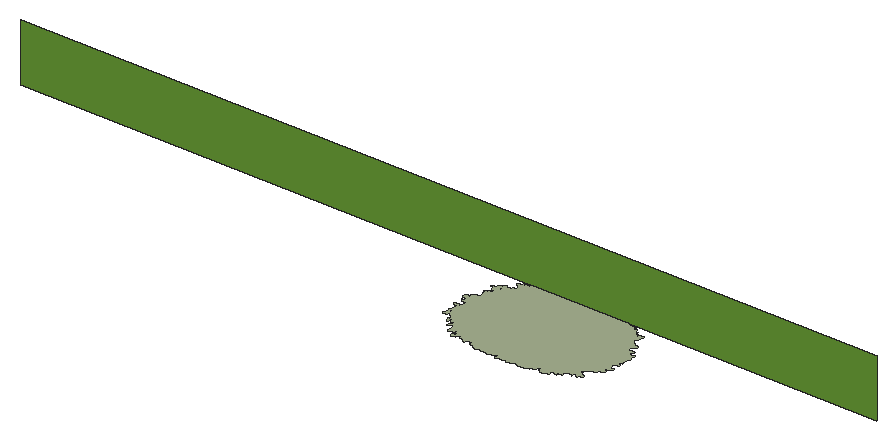
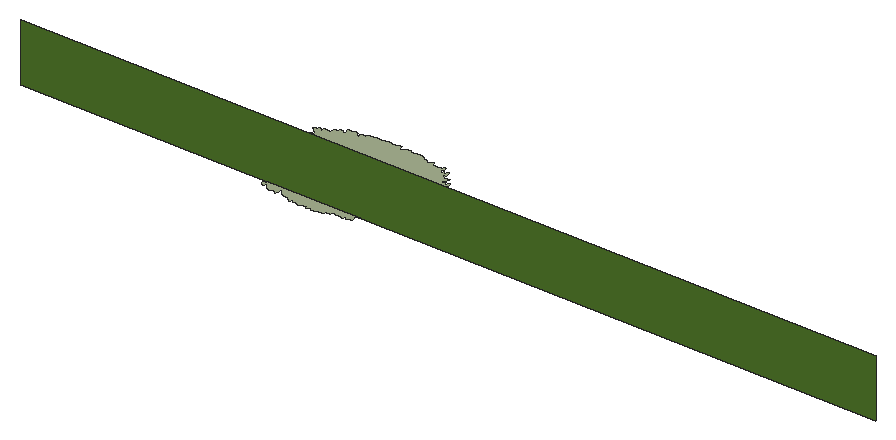
# SketchUp Ruby script. Lengths in inches.
U = 1.inch
M = Sketchup.active_model
def pt(a) = Geom::Point3d.new(a.map { |v| v * U })
def face(e, loops, mat)
  f = e.add_face(loops[0].map { |a| pt(a) })
  loops[1..].each { |l| e.add_face(l.map { |a| pt(a) }).erase! }
  f.material = f.back_material = mat if mat
  f
end
# faces: each face lists its corners as indices into pts; further lists are holes
def faces(e, pts, list, mat = nil) = list.each { |f| face(e, (f[0].is_a?(Array) ? f : [f]).map { |l| l.map { |i| pts[i] } }, mat) }
# xy, xz, yz: faces in a plane at the given z, y or x. An outline is a flat list of corners, or four numbers for a rectangle; further outlines are holes
def ring(l) = l.size == 4 ? [[l[0], l[1]], [l[2], l[1]], [l[2], l[3]], [l[0], l[3]]] : l.each_slice(2).to_a
def flat(e, list, mat, &to3) = list.each { |f| face(e, (f[0].is_a?(Array) ? f : [f]).map { |l| ring(l).map { |u, v| to3.(u, v) } }, mat) }
def xy(e, z, list, mat = nil) = flat(e, list, mat) { |x, y| [x, y, z] }
def xz(e, y, list, mat = nil) = flat(e, list, mat) { |x, z| [x, y, z] }
def yz(e, x, list, mat = nil) = flat(e, list, mat) { |y, z| [x, y, z] }
def lines(e, pts, list) = list.each { |a, b| e.add_line(pt(pts[a]), pt(pts[b])) }
# prism: a flat outline (further loops are holes) pulled along v
def prism(e, loops, v, mat = nil)
  f = face(e, loops, mat); d = Geom::Vector3d.new(v.map { |x| x * U })
  f.pushpull(f.normal.samedirection?(d) ? d.length : -d.length)
end
def box(e, o, s, mat = nil) = prism(e, [[o, [o[0] + s[0], o[1], o[2]], [o[0] + s[0], o[1] + s[1], o[2]], [o[0], o[1] + s[1], o[2]]]], [0, 0, s[2]], mat)
def at(x, y, z, deg = 0) = Geom::Transformation.translation(pt([x, y, z])) * Geom::Transformation.rotation(ORIGIN, Z_AXIS, deg.degrees)
def axes(o, x, y, z) = Geom::Transformation.new([*x, 0, *y, 0, *z, 0, *pt(o).to_a, 1])
def part(name) = M.definitions.add(name)
# library, detail: a bought-in or finely detailed component or shape, given as its bounding box
def library(name, o, s) = part(name).tap { |d| box(d.entities, o, s) }
def detail(e, o, s) = box(e.add_group.entities, o, s)
def put(e, d, t, mat = nil) = e.add_instance(d, t).tap { |i| i.material = mat if mat }
def group(e, t, mat = nil) = e.add_group.tap { |g| g.transformation = t; g.material = mat if mat }.entities
root = M.entities
M.materials.add("Boxwoodplan").color = [166, 177, 144]
M.materials.add("[Grass Dark Green]").color = [106, 157, 55]
xy(root,9.058,[[[215.792,67.129,215.681,67.133,215.586,67.159,215.53,67.215,215.528,67.317,215.554,67.382,215.618,67.445,215.667,67.509,215.725,67.606,215.539,67.635,215.449,67.644,215.469,67.732,215.555,67.79,215.586,67.8,215.581,67.846,215.492,67.877,215.376,67.837,215.279,67.706,215.136,67.551,214.975,67.464,214.87,67.441,214.809,67.416,214.793,67.373,214.649,67.281,214.455,67.251,214.366,67.26,214.286,67.306,214.286,67.328,214.331,67.359,214.422,67.437,214.49,67.483,214.401,67.498,214.288,67.48,214.168,67.436,214.072,67.445,213.975,67.454,213.878,67.447,213.751,67.403,213.551,67.356,213.462,67.349,213.424,67.443,213.416,67.465,213.349,67.473,213.26,67.454,213.091,67.336,212.891,67.328,212.661,67.353,212.494,67.446,212.353,67.61,212.536,67.702,212.436,67.756,212.3,67.772,212.174,67.749,212.102,67.697,212.021,67.672,211.905,67.738,211.863,67.806,211.951,67.847,211.977,67.907,211.982,67.957,211.941,68.009,211.869,68.085,211.783,68.117,211.696,68.064,211.63,68.038,211.574,68.08,211.557,68.103,211.533,68.121,211.504,68.111,211.424,68.058,211.353,68.01,211.277,67.923,211.265,67.79,211.194,67.749,211.144,67.723,211.084,67.725,210.985,67.746,210.898,67.793,210.854,67.861,210.846,67.951,210.855,68.018,210.868,68.04,210.849,68.08,210.635,68.1,210.703,68.135,210.677,68.136,210.584,68.13,210.414,68.146,210.337,68.173,210.32,68.206,210.335,68.224,210.46,68.314,210.458,68.371,210.373,68.393,210.214,68.39,210.083,68.319,209.986,68.233,209.911,68.199,209.864,68.172,209.863,68.154,209.899,68.101,209.883,68.046,209.813,68.081,209.749,68.121,209.688,68.072,209.666,68.017,209.634,67.904,209.587,67.855,209.514,67.822,209.423,67.816,209.353,67.841,209.334,67.874,209.341,67.892,209.362,67.932,209.384,67.991,209.353,68.048,209.252,68.149,209.366,68.229,209.427,68.269,209.507,68.285,209.574,68.315,209.629,68.37,209.714,68.476,209.642,68.503,209.5625,68.511,209.43,68.53,209.392,68.565,209.399,68.584,209.474,68.62,209.636,68.657,209.678,68.709,209.673,68.748,209.647,68.764,209.497,68.711,209.451,68.732,209.452,68.752,209.475,68.814,209.314,68.825,209.233,68.833,209.179,68.826,209.172,68.806,209.156,68.71,209.141,68.642,209.099,68.591,209.052,68.578,209.033,68.594,208.974,68.639,208.929,68.757,208.89,68.783,208.863,68.784,208.809,68.777,208.802,68.757,208.8,68.641,208.746,68.523,208.685,68.449,208.605,68.419,208.526,68.422,208.48,68.448,208.447,68.506,208.447,68.564,208.501,68.677,208.615,68.784,208.635,68.803,208.622,68.823,208.595,68.829,208.515,68.847,208.434,68.86,208.407,68.875,208.414,68.895,208.434,68.914,208.583,68.982,208.745,69.005,208.787,69.108,208.76,69.169,208.713,69.191,208.686,69.187,208.523,69.168,208.482,69.2,208.489,69.22,208.516,69.279,208.674,69.334,208.846,69.403,208.894,69.442,208.881,69.463,208.784,69.436,208.613,69.417,208.469,69.372,208.38,69.386,208.353,69.392,208.359,69.412,208.38,69.426,208.435,69.47,208.407,69.507,208.38,69.503,208.297,69.511,208.242,69.56,208.228,69.601,208.201,69.597,208.118,69.575,207.961,69.489,207.812,69.413,207.738,69.38,207.683,69.392,207.696,69.412,207.715,69.452,207.742,69.469,207.766,69.55,207.816,69.65,207.848,69.759,207.899,69.812,207.972,69.852,208.016,69.972,208.038,70.112,208.058,70.227,208.054,70.285,208.009,70.321,207.928,70.335,207.842,70.335,207.768,70.31,207.758,70.245,207.759,70.184,207.726,70.124,207.638,70.087,207.581,70.096,207.543,70.155,207.532,70.216,207.506,70.337,207.501,70.4,207.46,70.453,207.433,70.475,207.395,70.491,207.336,70.479,207.302,70.46,207.3,70.428,207.292,70.366,207.295,70.229,207.32,70.167,207.312,70.103,207.261,70.038,207.213,70.01,207.175,69.998,207.137,70.003,207.095,70.011,207.077,70.039,207.073,70.166,207.094,70.223,207.139,70.276,207.155,70.306,207.147,70.334,207.09,70.34,207.008,70.346,206.971,70.362,206.948,70.39,206.945,70.453,206.96,70.483,206.995,70.499,207.167,70.472,207.246,70.497,207.295,70.526,207.356,70.573,207.369,70.636,207.346,70.662,207.302,70.664,207.225,70.67,207.133,70.681,207.032,70.717,207.013,70.746,207.019,70.76,207.038,70.763,207.098,70.775,207.273,70.761,207.363,70.787,207.375,70.844,207.349,70.907,207.277,70.946,207.198,70.953,207.085,70.946,206.985,70.921,206.902,70.939,206.898,70.968,206.918,70.997,206.965,71.054,207.031,71.11,207.084,71.19,207.076,71.224,207.031,71.241,206.966,71.24,206.848,71.14,206.808,71.141,206.774,71.161,206.796,71.22,206.812,71.287,206.769,71.35,206.729,71.366,206.709,71.367,206.703,71.352,206.707,71.306,206.704,71.164,206.663,71.102,206.624,71.108,206.589,71.131,206.491,71.262,206.467,71.327,206.442,71.355,206.427,71.344,206.371,71.293,206.336,71.234,206.356,71.103,206.361,71.037,206.341,70.971,206.291,70.962,206.257,70.978,206.247,71.023,206.267,71.155,206.276,71.233,206.276,71.27,206.261,71.282,206.246,71.272,206.167,71.237,206.127,71.183,206.118,71.12,206.079,71.077,205.942,70.987,205.902,70.977,205.858,70.986,205.778,71.026,205.758,71.056,205.762,71.089,205.795,71.151,205.892,71.237,205.982,71.263,206.072,71.263,206.167,71.267,206.106,71.318,205.955,71.404,205.938,71.466,205.991,71.503,206.083,71.573,206.202,71.635,206.32,71.709,206.356,71.723,206.382,71.746,206.408,71.789,206.411,71.882,206.444,72.003,206.445,72.065,206.424,72.086,206.402,72.095,206.339,72.109,206.306,72.104,206.302,72.088,206.314,71.996,206.272,71.934,206.224,71.899,206.147,71.871,206.076,71.858,205.915,71.833,205.88,71.839,205.867,71.853,205.867,71.86,205.876,71.901,205.893,71.947,205.935,71.995,206.004,72.042,206.063,72.063,206.121,72.065,206.16,72.068,206.18,72.075,206.203,72.096,206.198,72.121,206.144,72.151,206.076,72.207,206.044,72.264,206.04,72.331,206.053,72.382,206.105,72.426,206.131,72.432,206.142,72.425,206.162,72.411,206.205,72.35,206.254,72.304,206.382,72.226,206.456,72.192,206.491,72.177,206.511,72.184,206.535,72.206,206.542,72.222,206.553,72.263,206.538,72.32,206.495,72.366,206.463,72.389,206.429,72.401,206.369,72.401,206.295,72.404,206.252,72.446,206.166,72.519,206.107,72.569,206.068,72.617,206.069,72.646,206.093,72.671,206.149,72.698,206.184,72.703,206.225,72.7,206.285,72.679,206.347,72.677,206.383,72.684,206.417,72.726,206.466,72.757,206.525,72.764,206.596,72.764,206.75,72.771,206.89,72.792,206.923,72.808,206.924,72.826,206.918,72.868,206.906,72.913,206.917,72.957,206.947,73.06,206.934,73.083,206.911,73.097,206.854,73.126,206.801,73.164,206.728,73.192,206.655,73.195,206.605,73.184,206.584,73.17,206.559,73.119,206.564,73.098,206.575,73.093,206.599,73.088,206.75,73.076,206.776,73.071,206.781,73.0625,206.772,73.046,206.732,73.007,206.687,72.964,206.622,72.928,206.56,72.884,206.488,72.849,206.451,72.852,206.431,72.863,206.406,72.9,206.399,72.995,206.382,73.02,206.4,73.034,206.406,73.077,206.4,73.088,206.389,73.088,206.374,73.087,206.348,73.083,206.316,73.076,206.298,73.065,206.217,72.97,206.185,72.915,206.154,72.892,206.131,72.895,206.105,72.916,206.096,72.932,206.09,72.973,206.119,73.057,206.124,73.102,206.115,73.13,206.095,73.137,206.057,73.128,206.037,73.114,205.991,73.064,205.869,72.957,205.833,72.932,205.807,72.927,205.77,72.935,205.758,72.951,205.849,73.057,205.912,73.102,205.926,73.129,205.925,73.145,205.916,73.152,205.905,73.148,205.89,73.143,205.859,73.131,205.775,73.108,205.608,73.089,205.535,73.096,205.487,73.121,205.465,73.149,205.464,73.165,205.481,73.217,205.529,73.264,205.589,73.281,205.66,73.284,205.734,73.266,205.862,73.223,205.948,73.197,205.959,73.201,205.959,73.22,205.95,73.239,205.925,73.287,205.924,73.342,205.931,73.407,205.943,73.437,205.96,73.45,206.009,73.413,206.048,73.363,206.075,73.317,206.085,73.255,206.097,73.204,206.112,73.176,206.135,73.175,206.27,73.157,206.343,73.144,206.378,73.14,206.396,73.154,206.411,73.202,206.356,73.244,206.297,73.309,206.28,73.335,206.28,73.352,206.314,73.46,206.344,73.483,206.371,73.489,206.386,73.477,206.395,73.459,206.424,73.414,206.435,73.39,206.447,73.391,206.468,73.404,206.548,73.482,206.565,73.528,206.566,73.579,206.552,73.611,206.531,73.623,206.468,73.646,206.428,73.666,206.42,73.687,206.436,73.736,206.492,73.773,206.526,73.795,206.539,73.816,206.547,73.869,206.545,73.916,206.45,73.992,206.306,74.014,206.244,74.031,206.209,74.013,206.181,74.014,206.112,74.031,206.093,74.058,206.102,74.082,206.228,74.185,206.222,74.217,206.2,74.233,206.155,74.225,206.126,74.216,206,74.154,205.96,74.107,205.911,74.063,205.842,74.049,205.814,74.05,205.767,74.102,205.795,74.126,205.8125,74.165,205.844,74.188,205.938,74.22,205.983,74.25,205.972,74.281,205.959,74.283,205.949,74.276,205.923,74.27,205.884,74.273,205.749,74.284,205.602,74.3125,205.578,74.327,205.584,74.347,205.609,74.375,205.822,74.435,205.885,74.434,205.946,74.419,206.006,74.391,206.033,74.393,206.039,74.403,206.088,74.48,206.112,74.495,206.118,74.515,206.118,74.583,206.107,74.593,206.094,74.591,206.036,74.591,205.979,74.585,205.932,74.568,205.908,74.576,205.887,74.596,205.862,74.63,205.842,74.718,205.853,74.806,205.883,74.848,205.889,74.88,205.902,74.923,205.939,74.944,205.935,74.99,205.913,75.026,205.824,75.003,205.806,74.969,205.807,74.95,205.81,74.886,205.73,74.839,205.589,74.745,205.433,74.7,205.349,74.725,205.307,74.778,205.298,74.904,205.426,74.99,205.509,75.003,205.552,75.027,205.576,75.061,205.575,75.081,205.489,75.112,205.416,75.138,205.354,75.194,205.389,75.249,205.465,75.278,205.561,75.312,205.626,75.311,205.805,75.267,205.897,75.246,205.982,75.25,206.033,75.269,206.039,75.289,206.023,75.355,205.962,75.407,205.917,75.415,205.805,75.485,205.758,75.527,205.744,75.564,205.737,75.617,205.737,75.644,205.75,75.659,205.792,75.695,205.843,75.709,205.957,75.741,205.988,75.751,206.028,75.75,206.078,75.746,206.091,75.733,206.106,75.703,206.12,75.689,206.13,75.689,206.158,75.692,206.174,75.704,206.195,75.754,206.223,75.787,206.239,75.81,206.242,75.835,206.258,75.86,206.278,75.872,206.326,75.884,206.365,75.877,206.386,75.833,206.39,75.781,206.407,75.755,206.428,75.754,206.47,75.796,206.495,75.838,206.509,75.942,206.525,75.968,206.557,75.975,206.589,75.974,206.608,75.963,206.629,75.94,206.661,75.94,206.714,75.961,206.758,76.007,206.772,76.032,206.761,76.046,206.821,76.043,206.85,76.046,206.866,76.066,206.871,76.114,206.905,76.155,206.939,76.2,206.885,76.243,206.818,76.272,206.781,76.271,206.748,76.261,206.706,76.249,206.664,76.255,206.642,76.271,206.621,76.295,206.598,76.397,206.611,76.423,206.616,76.439,206.626,76.443,206.731,76.463,206.777,76.472,206.795,76.483,206.785,76.486,206.699,76.514,206.633,76.526,206.605,76.519,206.57,76.52,206.534,76.52,206.498,76.532,206.46,76.582,206.442,76.611,206.442,76.642,206.457,76.663,206.486,76.678,206.517,76.697,206.525,76.725,206.555,76.782,206.582,76.836,206.588,76.89,206.581,76.917,206.541,76.928,206.463,76.954,206.29,77.001,206.254,77.018,206.237,77.042,206.273,77.097,206.317,77.131,206.363,77.159,206.418,77.178,206.47,77.1875,206.523,77.184,206.578,77.16,206.633,77.162,206.66,77.167,206.673,77.187,206.69,77.228,206.727,77.264,206.748,77.282,206.774,77.284,206.843,77.267,206.905,77.256,206.931,77.253,206.955,77.268,207.042,77.336,207.129,77.401,207.183,77.498,207.179,77.542,207.138,77.579,207.021,77.617,206.895,77.647,206.809,77.719,206.751,77.755,206.682,77.776,206.655,77.788,206.641,77.808,206.663,77.855,206.711,77.896,206.709,77.981,206.659,78.06,206.529,78.116,206.241,78.212,206.22,78.246,206.292,78.31,206.413,78.362,206.518,78.367,206.575,78.353,206.619,78.327,206.668,78.317,206.721,78.326,206.782,78.337,206.811,78.368,206.826,78.448,206.843,78.483,206.897,78.482,206.954,78.471,207.002,78.451,207.069,78.392,207.093,78.358,207.107,78.318,207.108,78.249,207.114,78.245,207.123,78.249,207.15,78.262,207.201,78.268,207.29,78.271,207.37,78.235,207.404,78.17,207.429,78.092,207.499,78.047,207.539,78.035,207.557,78.034,207.584,78.043,207.679,78.05,207.696,78.055,207.676,78.071,207.613,78.095,207.561,78.099,207.523,78.118,207.504,78.152,207.501,78.164,207.504,78.184,207.519,78.191,207.554,78.192,207.596,78.185,207.702,78.156,207.817,78.152,207.869,78.159,207.887,78.162,207.913,78.173,207.869,78.203,207.828,78.213,207.742,78.228,207.684,78.242,207.643,78.244,207.621,78.248,207.596,78.263,207.544,78.289,207.497,78.315,207.475,78.348,207.485,78.404,207.514,78.442,207.555,78.471,207.515,78.502,207.46,78.517,207.417,78.52,207.362,78.528,207.331,78.555,207.313,78.591,207.299,78.6,207.27,78.599,207.154,78.571,207.102,78.557,207.053,78.559,207.005,78.562,206.956,78.578,206.908,78.595,206.868,78.602,206.782,78.65,206.807,78.662,206.809,78.669,206.82,78.709,206.836,78.745,206.862,78.782,206.893,78.814,206.937,78.839,206.99,78.862,207.035,78.873,207.141,78.867,207.218,78.862,207.251,78.858,207.262,78.857,207.262,78.87,207.254,78.912,207.233,78.956,207.197,78.995,207.154,79.026,207.121,79.073,207.123,79.096,207.134,79.117,207.181,79.147,207.233,79.17,207.26,79.169,207.286,79.163,207.34,79.148,207.408,79.142,207.455,79.127,207.479,79.114,207.497,79.095,207.541,79.055,207.58,79.02,207.625,78.989,207.681,78.976,207.735,78.981,207.78,79.01,207.812,79.046,207.861,79.084,207.887,79.083,207.909,79.069,207.95,79.027,207.997,78.994,208.125,79.019,208.199,79.037,208.24,79.065,208.246,79.085,208.225,79.102,208.174,79.124,208.164,79.147,208.172,79.169,208.188,79.214,208.195,79.273,208.199,79.299,208.222,79.315,208.249,79.316,208.279,79.308,208.321,79.288,208.455,79.248,208.516,79.226,208.555,79.193,208.582,79.153,208.597,79.13,208.604,79.123,208.613,79.126,208.621,79.131,208.654,79.176,208.66,79.212,208.65,79.315,208.628,79.362,208.604,79.397,208.569,79.436,208.559,79.466,208.57,79.477,208.581,79.475,208.603,79.476,208.602,79.484,208.607,79.508,208.6,79.549,208.585,79.705,208.587,79.782,208.472,79.802,208.375,79.804,208.3125,79.8125,208.295,79.819,208.281,79.83,208.294,79.839,208.407,79.882,208.441,79.911,208.44,79.924,208.417,79.948,208.381,79.952,208.328,79.94,208.28,79.918,208.263,79.919,208.248,79.945,208.274,80.028,208.277,80.069,208.276,80.082,208.252,80.103,208.163,80.085,208.05,80.088,207.941,80.105,207.88,80.185,207.878,80.213,207.916,80.25,208.012,80.303,208.061,80.33,208.115,80.335,208.24,80.332,208.331,80.337,208.391,80.346,208.431,80.384,208.471,80.418,208.479,80.461,208.505,80.5,208.561,80.513,208.598,80.509,208.641,80.475,208.652,80.389,208.659,80.3,208.683,80.257,208.738,80.231,208.83,80.212,208.885,80.234,208.903,80.276,208.88,80.319,208.833,80.355,208.777,80.442,208.813,80.521,208.887,80.603,208.906,80.606,208.93,80.576,208.949,80.528,209.023,80.447,209.051,80.421,209.042,80.475,209.024,80.57,209.08,80.587,209.141,80.582,209.268,80.578,209.381,80.575,209.503,80.557,209.521,80.557,209.509,80.587,209.458,80.629,209.328,80.681,209.29,80.689,209.267,80.735,209.269,80.826,209.304,80.871,209.353,80.896,209.469,80.901,209.566,80.91,209.661,80.977,209.787,80.982,209.903,80.971,209.999,80.953,210.12,80.946,210.163,80.991,210.176,81.038,210.219,81.133,210.308,81.187,210.428,81.244,210.44,81.26,210.423,81.294,210.382,81.332,210.275,81.413,210.207,81.487,210.149,81.528,210.092,81.57,210.123,81.577,210.122,81.591,210.117,81.612,210.106,81.679,210.109,81.709,210.144,81.744,210.227,81.785,210.31,81.821,210.348,81.827,210.404,81.826,210.491,81.816,210.514,81.808,210.538,81.81,210.57,81.843,210.622,81.918,210.658,81.932,210.715,81.936,210.817,81.93,210.913,81.898,210.945,81.877,210.974,81.835,210.975,81.765,210.978,81.736,210.983,81.715,211.006,81.704,211.059,81.715,211.104,81.745,211.166,81.798,211.191,81.822,211.212,81.834,211.225,81.85,211.14,81.897,211.102,81.913,211.059,81.956,211.034,82.036,211.035,82.067,211.093,82.083,211.285,82.055,211.382,82.039,211.417,82.026,211.417,81.98,211.427,81.952,211.487,81.948,211.591,81.962,211.693,81.975,211.735,81.971,211.782,81.957,211.809,81.934,211.834,81.933,211.859,81.943,212.003,81.972,212.044,81.981,212.096,81.987,212.132,81.984,212.177,81.957,212.207,81.886,212.233,81.863,212.278,81.844,212.318,81.833,212.358,81.808,212.41,81.753,212.464,81.696,212.451,81.619,212.444,81.545,212.458,81.515,212.489,81.485,212.516,81.461,212.563,81.453,212.599,81.45,212.644,81.481,212.657,81.512,212.658,81.553,212.646,81.628,212.683,81.787,212.672,81.817,212.654,81.829,212.63,81.833,212.591,81.834,212.539,81.828,212.503,81.826,212.456,81.835,212.431,81.858,212.438,81.88,212.466,81.896,212.505,81.91,212.55,81.937,212.575,82.013,212.579,82.178,212.579,82.21,212.602,82.228,212.628,82.233,212.727,82.222,212.926,82.201,213.017,82.19,213.106,82.169,213.193,82.153,213.244,82.147,213.239,82.355,213.307,82.427,213.392,82.486,213.446,82.477,213.474,82.441,213.522,82.37,213.545,82.297,213.553,82.26,213.551,82.241,213.578,82.206,213.683,82.173,213.735,82.173,213.774,82.204,213.777,82.279,213.674,82.36,213.596,82.419,213.608,82.453,213.652,82.49,213.746,82.541,213.796,82.55,213.877,82.538,213.981,82.537,214.004,82.615,214.214,82.643,214.314,82.661,214.422,82.647,214.501,82.578,214.534,82.543,214.561,82.541,214.601,82.568,214.599,82.643,214.59,82.685,214.603,82.72,214.653,82.729,214.708,82.715,214.779,82.621,214.8,82.548,214.833,82.513,214.882,82.498,214.933,82.503,214.979,82.53,215.067,82.613,215.148,82.668,215.25,82.715,215.298,82.7,215.312,82.663,215.26,82.592,215.234,82.557,215.242,82.515,215.331,82.457,215.431,82.443,215.481,82.452,215.531,82.498,215.609,82.566,215.724,82.581,215.839,82.553,215.87,82.523,215.947,82.492,216.047,82.511,216.129,82.565,216.129,82.678,216.186,82.721,216.299,82.745,216.404,82.74,216.485,82.681,216.631,82.66,216.685,82.651,216.691,82.614,216.617,82.546,216.584,82.473,216.596,82.437,216.668,82.396,216.77,82.401,216.823,82.433,216.843,82.472,216.863,82.544,216.912,82.567,216.936,82.579,216.987,82.579,217.09,82.541,217.133,82.47,217.219,82.417,217.349,82.447,217.384,82.478,217.39,82.52,217.43,82.603,217.537,82.622,217.567,82.592,217.573,82.55,217.52,82.466,217.472,82.448,217.445,82.413,217.505,82.349,217.636,82.337,217.727,82.373,217.794,82.444,217.819,82.45,217.828,82.433,217.846,82.392,217.87,82.357,217.859,82.301,217.839,82.257,217.857,82.222,217.946,82.179,218.054,82.184,218.109,82.203,218.16,82.258,218.177,82.273,218.179,82.255,218.166,82.212,218.093,82.132,218.059,82.102,218.07,82.066,218.117,82.047,218.175,82.048,218.271,82.088,218.353,82.146,218.573,82.225,218.595,82.153,218.618,82.123,218.669,82.118,218.785,82.11,218.909,82.084,218.924,82.013,218.947,81.983,218.993,81.964,219.016,81.93,219.002,81.892,218.975,81.795,219.092,81.773,219.138,81.755,219.148,81.72,219.074,81.65,219.06,81.613,219.076,81.579,219.152,81.527,219.255,81.5,219.356,81.496,219.468,81.563,219.51,81.639,219.452,81.71,219.419,81.779,219.439,81.885,219.448,81.922,219.419,81.956,219.415,81.992,219.457,82.018,219.558,82.022,219.547,82.122,219.505,82.274,219.555,82.287,219.62,82.275,219.673,82.256,219.704,82.199,219.654,82.131,219.658,82.095,219.704,82.076,219.812,82.076,219.942,82.111,220.449,82.178,220.495,82.168,220.541,82.145,220.587,82.121,220.621,82.097,220.652,82.027,220.635,81.935,220.839,81.949,220.904,81.943,220.989,81.911,221.026,81.805,221.011,81.757,220.995,81.724,220.954,81.717,220.784,81.749,220.72,81.755,220.677,81.755,220.657,81.749,220.654,81.733,220.682,81.685,220.723,81.666,220.77,81.666,220.943,81.681,221.012,81.683,221.096,81.648,221.133,81.609,221.164,81.546,221.232,81.437,221.311,81.398,221.396,81.394,221.427,81.435,221.421,81.518,221.403,81.571,221.41,81.637,221.451,81.687,221.552,81.719,221.661,81.732,221.75,81.701,221.798,81.659,221.832,81.597,221.833,81.551,221.771,81.495,221.705,81.482,221.664,81.471,221.632,81.437,221.636,81.407,221.685,81.389,221.783,81.363,221.854,81.339,221.874,81.306,221.862,81.275,221.808,81.247,221.721,81.24,221.559,81.233,221.472,81.222,221.383,81.256,221.319,81.269,221.237,81.251,221.181,81.208,221.179,81.143,221.237,81.103,221.324,81.081,221.41,81.066,221.457,81.066,221.491,81.046,221.512,81.003,221.495,80.938,221.46,80.89,221.432,80.866,221.387,80.854,221.245,80.834,221.225,80.829,221.216,80.784,221.22,80.751,221.265,80.732,221.332,80.731,221.373,80.731,221.423,80.746,221.486,80.778,221.5,80.712,221.471,80.665,221.464,80.635,221.503,80.617,221.564,80.622,221.646,80.67,221.702,80.711,221.73,80.736,221.768,80.721,221.832,80.704,221.901,80.651,221.897,80.603,221.854,80.537,221.821,80.472,221.839,80.448,221.886,80.445,221.962,80.456,222.044,80.495,222.083,80.554,222.155,80.597,222.215,80.609,222.252,80.601,222.27,80.577,222.273,80.548,222.256,80.521,222.228,80.497,222.23,80.483,222.251,80.481,222.423,80.499,222.504,80.51,222.571,80.552,222.613,80.589,222.692,80.614,222.789,80.619,222.812,80.595,222.815,80.566,222.655,80.349,222.67,80.304,222.727,80.251,222.81,80.237,222.899,80.255,222.967,80.283,223.052,80.305,223.117,80.213,223.153,79.999,223.155,79.985,223.191,79.974,223.275,79.996,223.286,79.918,223.31,79.871,223.386,79.861,223.523,79.896,223.591,79.893,223.606,79.839,223.538,79.619,223.527,79.567,223.55,79.514,223.616,79.486,223.684,79.496,223.82,79.523,223.84,79.419,223.835,79.316,223.957,79.247,224.09,79.216,224.12,79.318,224.11,79.421,224.087,79.474,224.115,79.525,224.184,79.535,224.223,79.482,224.245,79.429,224.293,79.395,224.37,79.418,224.424,79.467,224.448,79.583,224.452,79.636,224.513,79.659,224.57,79.631,224.6,79.577,224.575,79.455,224.46,79.375,224.407,79.339,224.386,79.282,224.366,79.231,224.389,79.186,224.521,79.161,224.577,79.134,224.582,79.083,224.509,78.997,224.544,78.895,224.573,78.844,224.561,78.794,224.427,78.768,224.326,78.729,224.222,78.658,224.171,78.623,224.105,78.626,224.041,78.659,224.009,78.667,223.983,78.643,224.027,78.549,224.146,78.483,224.193,78.445,224.19,78.396,224.275,78.32,224.441,78.132,224.573,78.05,224.636,78.035,224.673,77.992,224.658,77.898,224.774,77.834,224.711,77.749,224.691,77.697,224.689,77.673,224.72,77.661,224.857,77.679,224.992,77.755,225.122,77.768,225.247,77.734,225.25,77.687,225.184,77.66,225.158,77.644,225.172,77.62,225.25,77.599,225.322,77.596,225.354,77.595,225.367,77.571,225.279,77.482,225.113,77.322,225.089,77.232,225.085,77.187,225.057,77.142,224.964,77.067,224.836,77.038,224.711,77.043,224.602,77.082,224.533,77.076,224.506,77.004,224.533,76.894,224.504,76.787,224.386,76.72,224.414,76.62,224.552,76.642,224.724,76.833,224.951,76.815,225.027,76.605,225.072,76.595,225.154,76.618,225.241,76.723,225.379,76.735,225.417,76.635,225.367,76.574,225.352,76.539,225.429,76.501,225.568,76.531,225.6875,76.598,225.734,76.614,225.824,76.592,225.802,76.477,225.691,76.384,225.626,76.289,225.634,76.113,225.62,76.078,225.527,76.056,225.395,76.087,225.42,75.981,225.551,75.941,225.697,75.936,225.846,75.965,226.083,76.087,226.219,76.099,226.311,76.008,226.278,75.905,226.138,75.849,226.091,75.825,226.0625,75.766,226.166,75.675,226.317,75.515,226.284,75.414,226.168,75.359,226.132,75.335,226.17,75.274,226.314,75.269,226.444,75.247,226.456,75.145,226.383,75.089,226.25,75.078,226.125,75.041,226.082,74.942,226.25,74.761,226.143,74.568,226.146,74.388,226.2,74.176,226.244,74.078,226.112,74.051,225.989,74.008,225.895,73.931,225.868,73.869,225.979,73.801,226.231,73.744,226.308,73.662,226.329,73.559,226.287,73.467,226.172,73.394,225.711,73.234,225.713,73.141,225.757,73.048,225.811,72.954,225.8125,72.863,225.807,72.803,225.804,72.773,225.83,72.719,225.951,72.676,226.076,72.672,226.202,72.682,226.244,72.68,226.302,72.633,226.313,72.453,226.286,72.395,226.177,72.347,226.05,72.33,226.009,72.331,225.963,72.281,226.005,72.191,225.992,72.163,225.907,72.144,225.866,72.145,225.796,72.17,225.764,72.26,225.694,72.292,225.571,72.297,225.529,72.291,225.513,72.233,225.589,72.156,225.676,71.992,225.704,71.969,225.73,71.918,225.748,71.888,225.829,71.877,225.909,71.86,225.994,71.792,226.057,71.71,226.054,71.681,225.97,71.656,225.721,71.616,225.526,71.488,225.453,71.469,225.358,71.544,225.318,71.553,225.254,71.52,225.257,71.435,225.313,71.27,225.271,71.264,225.238,71.219,225.189,71.18,225.135,71.066,225.096,71.019,225.062,71,225.026,71.013,224.904,71.1,224.841,71.115,224.798,71.116,224.753,71.098,224.69,71.063,224.66,70.991,224.67,70.938,224.652,70.874,224.49,70.852,224.438,70.81,224.406,70.759,224.359,70.718,224.347,70.655,224.316,70.609,224.282,70.583,224.245,70.573,224.176,70.564,224.078,70.575,224.018,70.55,223.956,70.502,223.926,70.457,224.001,70.419,224.028,70.376,223.992,70.32,223.937,70.284,223.916,70.225,223.915,70.209,223.914,70.194,223.933,70.186,224.005,70.18,224.031,70.182,224.051,70.182,224.055,70.166,224.017,70.097,223.998,70.049,223.995,70.02,224.036,70.018,224.175,70.094,224.244,70.11,224.325,70.107,224.309,70.004,224.291,69.89,224.291,69.843,224.314,69.82,224.354,69.818,224.418,69.845,224.499,69.846,224.558,69.832,224.598,69.827,224.604,69.798,224.564,69.76,224.485,69.73,224.419,69.722,224.336,69.696,224.297,69.658,224.28,69.602,224.284,69.587,224.324,69.586,224.406,69.611,224.564,69.673,224.718,69.703,224.844,69.705,224.896,69.685,224.871,69.611,224.85,69.569,224.789,69.518,224.636,69.492,224.497,69.491,224.436,69.482,224.405,69.427,224.431,69.308,224.416,69.264,224.335,69.243,224.199,69.255,224.141,69.261,224.097,69.314,224.088,69.426,224.088,69.468,224.076,69.496,224.067,69.511,224.047,69.512,223.989,69.525,223.984,69.581,223.986,69.595,223.982,69.61,223.963,69.614,223.883,69.617,223.826,69.591,223.781,69.536,223.744,69.499,223.719,69.44,223.73,69.391,223.786,69.354,223.861,69.254,223.857,69.155,223.848,69.115,223.841,69.088,223.81,69.066,223.79,69.067,223.769,69.098,223.74,69.157,223.675,69.258,223.634,69.298,223.62,69.312,223.609,69.299,223.602,69.271,223.599,69.227,223.58,69.173,223.574,69.16,223.544,69.144,223.461,69.137,223.32,69.139,223.034,69.14,222.976,69.162,222.889,69.173,222.87,69.163,222.864,69.133,222.914,69.074,222.939,68.976,222.933,68.936,222.901,68.896,222.877,68.889,222.817,68.88,222.714,68.88,222.616,68.884,222.568,68.853,222.623,68.829,222.724,68.814,222.832,68.78,222.907,68.726,222.988,68.654,222.97,68.629,222.909,68.614,222.808,68.621,222.771,68.63,222.72,68.65,222.672,68.684,222.622,68.708,222.587,68.63,222.577,68.558,222.537,68.545,222.481,68.558,222.436,68.589,222.423,68.6,222.405,68.608,222.393,68.59,222.359,68.513,222.361,68.485,222.394,68.448,222.486,68.416,222.525,68.383,222.538,68.34,222.536,68.326,222.517,68.323,222.474,68.36,222.394,68.409,222.301,68.427,222.244,68.429,222.232,68.415,222.253,68.39,222.367,68.347,222.404,68.335,222.427,68.292,222.423,68.264,222.422,68.251,222.379,68.249,222.266,68.26,222.161,68.295,222.126,68.325,222.117,68.371,222.116,68.441,222.065,68.461,222.006,68.442,221.906,68.449,221.807,68.467,221.78,68.489,221.755,68.526,221.759,68.568,221.765,68.583,221.727,68.591,221.633,68.616,221.576,68.619,221.541,68.606,221.529,68.577,221.509,68.571,221.482,68.597,221.479,68.612,221.509,68.635,221.525,68.646,221.517,68.671,221.43,68.729,221.393,68.752,221.374,68.756,221.333,68.736,221.293,68.716,221.273,68.71,221.262,68.681,221.285,68.59,221.38,68.587,221.419,68.582,221.449,68.541,221.442,68.513,221.436,68.499,221.444,68.471,221.555,68.434,221.643,68.396,221.704,68.338,221.721,68.3125,221.72,68.299,221.685,68.283,221.665,68.273,221.696,68.251,221.751,68.225,221.763,68.2,221.712,68.168,221.7,68.141,221.725,68.106,221.81,68.062,221.888,67.994,221.887,67.851,221.866,67.825,221.814,67.814,221.76,67.829,221.722,67.874,221.682,67.939,221.664,67.949,221.626,67.944,221.574,67.926,221.552,67.897,221.553,67.854,221.552,67.84,221.519,67.828,221.342,67.819,221.334,67.826,221.286,67.808,221.242,67.777,221.158,67.692,221.106,67.661,221.032,67.651,220.894,67.643,220.84,67.658,220.838,67.698,220.947,67.762,221.047,67.834,221.044,67.937,221.038,67.98,221.038,67.994,221.007,68.015,220.947,68.034,220.873,68.034,220.789,67.95,220.769,67.911,220.712,67.866,220.697,67.857,220.661,67.865,220.624,67.88,220.612,67.907,220.652,67.999,220.712,68.094,220.713,68.135,220.645,68.189,220.534,68.224,220.482,68.246,220.445,68.238,220.42,68.215,220.386,68.171,220.353,68.156,220.311,68.157,220.255,68.166,220.218,68.168,220.18,68.145,220.099,68.05,220.113,68.01,220.187,67.97,220.242,67.938,220.269,67.917,220.278,67.89,220.254,67.851,220.194,67.807,220.092,67.756,220.037,67.735,219.964,67.738,219.909,67.76,219.835,67.769,219.79,67.745,219.753,67.743,219.721,67.76,219.666,67.766,219.593,67.752,219.571,67.717,219.581,67.659,219.678,67.575,219.705,67.536,219.706,67.51,219.706,67.497,219.688,67.492,219.398,67.391,219.123,67.369,218.89,67.373,218.799,67.371,218.677,67.31,218.574,67.275,218.477,67.279,218.439,67.281,218.39,67.299,218.342,67.328,218.281,67.325,218.192,67.334,218.108,67.376,218.048,67.433,218.017,67.478,217.958,67.491,217.859,67.479,217.763,67.438,217.683,67.398,217.584,67.325,217.487,67.269,217.394,67.24,217.153,67.222,216.963,67.186,216.866,67.19,216.801,67.284,216.77,67.351,216.682,67.365,216.591,67.352,216.495,67.28,216.43,67.217,216.34,67.21,216.163,67.233,215.978,67.24,215.9,67.189],[206.3,74.415,206.342,74.419,206.362,74.422,206.388,74.431,206.4,74.474,206.401,74.513,206.408,74.597,206.4,74.631,206.388,74.643,206.388,74.658,206.345,74.635,206.289,74.612,206.269,74.606,206.253,74.59,206.232,74.557,206.222,74.52,206.224,74.476,206.243,74.437,206.262,74.421]]],"Boxwoodplan")
xz(root,80.932,[[144.115,9,253.103,16.375]],"[Grass Dark Green]")
